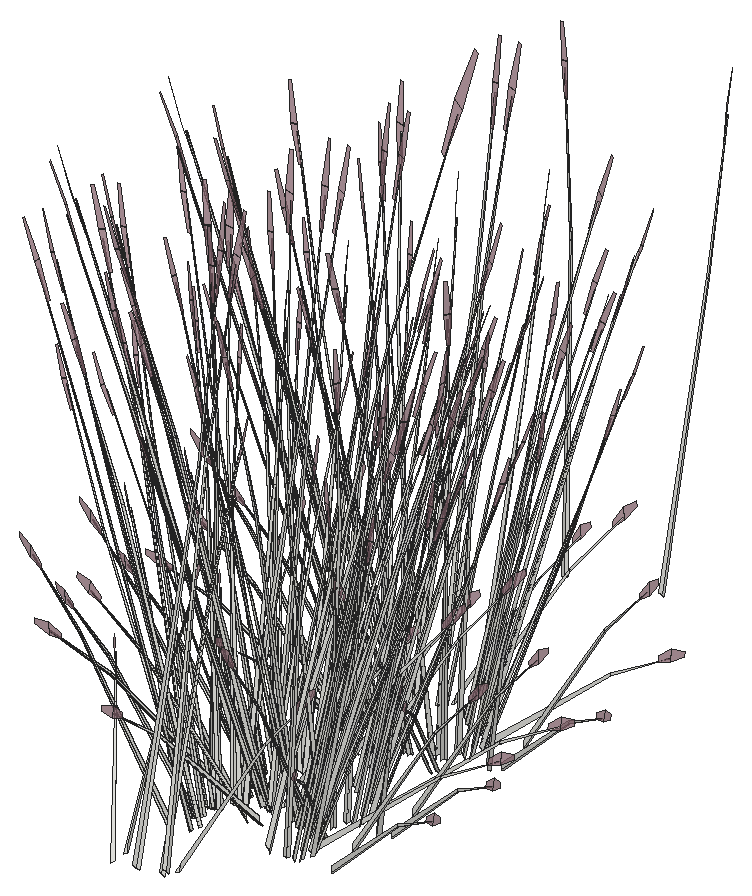
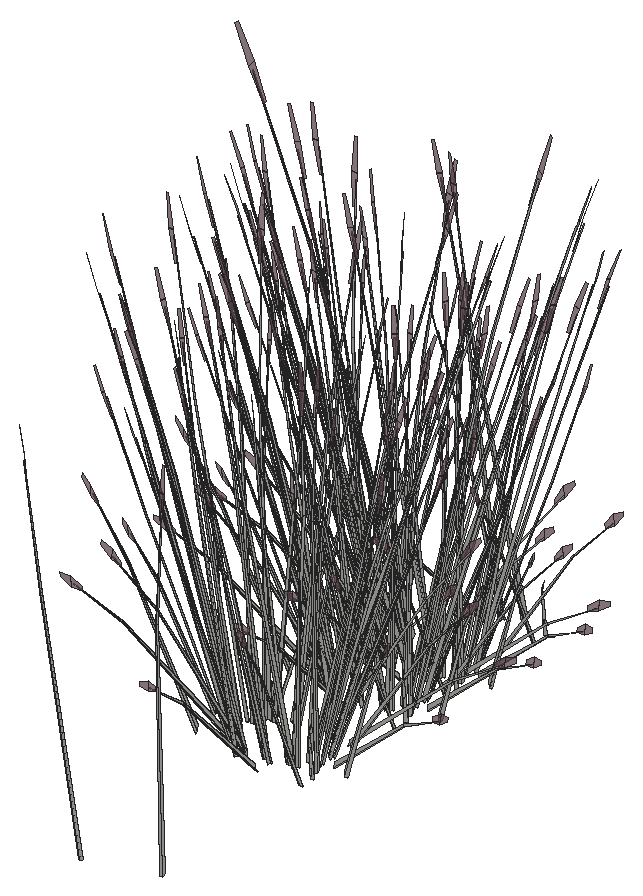
# SketchUp Ruby script. Lengths in inches.
U = 1.inch
M = Sketchup.active_model
def pt(a) = Geom::Point3d.new(a.map { |v| v * U })
def face(e, loops, mat)
  f = e.add_face(loops[0].map { |a| pt(a) })
  loops[1..].each { |l| e.add_face(l.map { |a| pt(a) }).erase! }
  f.material = f.back_material = mat if mat
  f
end
# faces: each face lists its corners as indices into pts; further lists are holes
def faces(e, pts, list, mat = nil) = list.each { |f| face(e, (f[0].is_a?(Array) ? f : [f]).map { |l| l.map { |i| pts[i] } }, mat) }
# xy, xz, yz: faces in a plane at the given z, y or x. An outline is a flat list of corners, or four numbers for a rectangle; further outlines are holes
def ring(l) = l.size == 4 ? [[l[0], l[1]], [l[2], l[1]], [l[2], l[3]], [l[0], l[3]]] : l.each_slice(2).to_a
def flat(e, list, mat, &to3) = list.each { |f| face(e, (f[0].is_a?(Array) ? f : [f]).map { |l| ring(l).map { |u, v| to3.(u, v) } }, mat) }
def xy(e, z, list, mat = nil) = flat(e, list, mat) { |x, y| [x, y, z] }
def xz(e, y, list, mat = nil) = flat(e, list, mat) { |x, z| [x, y, z] }
def yz(e, x, list, mat = nil) = flat(e, list, mat) { |y, z| [x, y, z] }
def lines(e, pts, list) = list.each { |a, b| e.add_line(pt(pts[a]), pt(pts[b])) }
# prism: a flat outline (further loops are holes) pulled along v
def prism(e, loops, v, mat = nil)
  f = face(e, loops, mat); d = Geom::Vector3d.new(v.map { |x| x * U })
  f.pushpull(f.normal.samedirection?(d) ? d.length : -d.length)
end
def box(e, o, s, mat = nil) = prism(e, [[o, [o[0] + s[0], o[1], o[2]], [o[0] + s[0], o[1] + s[1], o[2]], [o[0], o[1] + s[1], o[2]]]], [0, 0, s[2]], mat)
def at(x, y, z, deg = 0) = Geom::Transformation.translation(pt([x, y, z])) * Geom::Transformation.rotation(ORIGIN, Z_AXIS, deg.degrees)
def axes(o, x, y, z) = Geom::Transformation.new([*x, 0, *y, 0, *z, 0, *pt(o).to_a, 1])
def part(name) = M.definitions.add(name)
# library, detail: a bought-in or finely detailed component or shape, given as its bounding box
def library(name, o, s) = part(name).tap { |d| box(d.entities, o, s) }
def detail(e, o, s) = box(e.add_group.entities, o, s)
def put(e, d, t, mat = nil) = e.add_instance(d, t).tap { |i| i.material = mat if mat }
def group(e, t, mat = nil) = e.add_group.tap { |g| g.transformation = t; g.material = mat if mat }.entities
root = M.entities
M.materials.add("LightPink_Translucent").color = [144, 107, 117]
M.materials["LightPink_Translucent"].alpha = 0.75
c1 = part("blade")
p = [[2.15,0.21,22],[0,0.17,0],[0.09,0.45,0],[2.18,0.31,22],[2.29,0.31,22],[0.38,0.45,0],
  [2.48,0.24,33],[2.49,0.24,33],[2.48,0.22,33]]
faces(c1.entities,p,[[0,1,2,3],[4,5,2,3],[6,3,4,7],[8,0,3,6]])
c2 = part("seeds")
p = [[0.3,-0.1,1.38],[-0.01,-0.03,1.59],[-0.01,-0.03,0.03],[0.14,-0.07,-0.07],[0.29,-0.03,3],[0.15,0.01,3.11]]
faces(c2.entities,p,[[0,1,2,3],[1,0,4,5]],"LightPink_Translucent")
c3 = part("blade with seeds")
put(c3.entities,c1,at(0,0,0))
put(c3.entities,c2,axes([2.4,0.25,30.99],[1.5799,-0.05474,1.17369],[-0.12525,1.92788,0.29478],[-0.07173,-0.02425,1.56792]))
put(root,c3,axes([271.4375,361,127.375],[-0.6592,0.22175,0.0643],[-0.32265,-0.40436,0.50621],[0.06366,0.17825,0.77189]))
put(root,c3,axes([267.58,360.37,127.36],[-0.02224,0.12912,1.74944],[0.63107,0.44917,-0.27667],[-0.16521,0.21241,0.14031]))
put(root,c3,axes([269.6,360.08,128.04],[0.98321,0.03233,-0.13498],[-0.02687,0.61208,-0.74919],[-0.0683,0.23574,1.13838]))
put(root,c3,axes([275.86,367.16,127.73],[-0.77872,0.09325,0.35414],[-0.20563,-0.53305,-0.4572],[0.22316,-0.14318,0.87481]))
put(root,c3,axes([271.67,360.96,127.71],[-0.88151,-0.17057,0.53283],[0.30143,-0.56078,0.43934],[0.05297,0.22053,1.10256]))
put(root,c3,axes([276.5625,367.07,127.41],[0.61415,0.2744,0.0643],[-0.35756,0.39076,0.50621],[0.1969,-0.12633,0.77189]))
put(root,c3,axes([276.39,366.96,127.41],[0.22187,0.60049,0.48003],[-0.87033,0.10422,0.3958],[0.25651,-0.14123,0.9933]))
put(root,c3,axes([278.74,367.68,127.39],[0.12414,-0.09938,1.74944],[-0.15889,-0.60963,-0.27667],[0.31148,-0.11559,0.14031]))
put(root,c3,axes([271.98,369.52,127.26],[-0.13683,-0.09148,1.74944],[-0.91315,0.058,-0.27667],[-0.14574,-0.2188,0.14031]))
put(root,c3,axes([268.25,365.3,127.38],[0.06632,0.06511,1.77383],[-0.31973,0.58531,-0.16761],[-0.32381,0.00424,0.31391]))
put(root,c3,axes([267.51,361.69,127.35],[0.10149,-0.03939,1.77383],[0.83886,0.26202,-0.16761],[-0.01971,0.21816,0.31391]))
put(root,c3,axes([269.65,366.32,127.73],[0.50902,0.40851,0.35414],[-0.58122,0.38671,-0.4572],[-0.29531,-0.05884,0.87481]))
put(root,c3,axes([269.51,366.0625,127.71],[-0.0479,0.66354,-0.1216],[-0.90696,-0.01814,-0.67495],[-0.3493,-0.04609,1.02557]))
put(root,c3,axes([276.09,370.64,127.26],[-0.00864,-0.12985,1.74944],[-0.72937,-0.3753,-0.27667],[0.11277,-0.2275,0.14031]))
put(root,c3,axes([275.89,370.17,127.26],[-0.09085,0.04984,1.77383],[-0.89014,-0.16814,-0.16761],[-0.03222,-0.21748,0.31391]))
put(root,c3,axes([276.29,368.61,127.71],[-0.45012,-0.59081,-0.1216],[0.79888,-0.29033,-0.67495],[0.33665,-0.07795,1.02557]))
put(root,c3,axes([271.21,361.96,127.36],[0.1134,0.10507,1.74944],[0.91515,0.04128,-0.27667],[0.09203,0.23172,0.14031]))
put(root,c3,axes([271.05,369.22,127.26],[-0.01669,0.07821,1.77383],[-0.82314,0.28383,-0.16761],[-0.24223,-0.14508,0.31391]))
put(root,c3,axes([270.87,370.61,127.64],[0.99656,-0.1677,0.53763],[0.17295,0.65785,0.4433],[-0.23438,-0.19388,1.11249]))
put(root,c3,axes([273.12,370.73,127.28],[0.88151,0.17057,0.48003],[-0.30143,0.56078,0.3958],[-0.05297,-0.22053,0.9933]))
put(root,c3,axes([275.98,368.43,127.73],[-0.74348,-0.18202,0.35414],[0.21685,-0.53102,-0.4572],[0.29933,-0.04869,0.87481]))
put(root,c3,axes([273.35,370.6875,127.28],[0.6592,-0.22175,0.0643],[0.32265,0.40436,0.50621],[-0.06366,-0.17825,0.77189]))
put(root,c3,axes([268.2,367.46,127.41],[0.25275,-0.59491,0.48003],[0.83094,0.20343,0.3958],[-0.32677,0.03575,0.9933]))
put(root,c3,axes([268.14,367.3,127.41],[-0.32857,-0.44488,0.0643],[0.59916,-0.21775,0.50621],[-0.26412,0.04296,0.77189]))
put(root,c3,axes([271.09,370.75,127.28],[0.4066,-0.41448,0.0643],[0.57901,0.24131,0.50621],[-0.18719,-0.13288,0.77189]))
put(root,c3,axes([273.11,371.14,127.6],[-0.2697,0.50175,0.35414],[-0.78684,-0.14635,-0.4572],[-0.07215,-0.20201,0.87481]))
put(root,c3,axes([275.12,371.35,127.28],[0.63704,0.44518,0.48003],[-0.67652,0.38394,0.3958],[0.11751,-0.20886,0.9933]))
put(root,c3,axes([271.28,370.71,127.98],[-0.59706,0.6255,-0.13619],[-0.86465,-0.36036,-0.75594],[-0.30056,-0.17672,1.14864]))
put(root,c3,axes([275.36,371.4,127.28],[0.73517,0.0304,0.0643],[-0.02016,0.45906,0.50621],[0.07693,-0.17585,0.77189]))
put(root,c3,axes([276.66,368.6,127.41],[0.32857,0.44488,0.0643],[-0.59916,0.21775,0.50621],[0.26412,-0.04296,0.77189]))
put(root,c3,axes([274.81,371.71,127.6],[-0.60531,0.34352,0.35414],[-0.573,-0.39225,-0.4572],[0.08718,-0.19929,0.87481]))
put(root,c3,axes([276.59,368.4375,127.41],[-0.25275,0.59491,0.48003],[-0.83094,-0.20343,0.3958],[0.32677,-0.03575,0.9933]))
put(root,c3,axes([268.81,367.47,127.73],[0.74348,0.18202,0.35414],[-0.21685,0.53102,-0.4572],[-0.29933,0.04869,0.87481]))
put(root,c3,axes([268.99,370.53,127.26],[-0.19249,-0.00461,1.74944],[-0.61281,0.46055,-0.27667],[-0.32697,-0.0941,0.14031]))
put(root,c3,axes([271.22,371.23,127.6],[0.13817,0.52554,0.35414],[-0.78985,0.13877,-0.4572],[-0.21215,-0.1506,0.87481]))
put(root,c3,axes([268.85,371.57,127.64],[0.7388,-0.48151,0.53763],[0.63717,0.51135,0.4433],[-0.34662,-0.08882,1.11249]))
put(root,c3,axes([278.3,372.66,127.26],[-0.11685,-0.00496,1.77383],[-0.48522,-0.53096,-0.16761],[0.19486,-0.17458,0.31391]))
put(root,c3,axes([278.09,370.36,127.38],[-0.08089,-0.05712,1.77383],[0.17695,-0.61228,-0.16761],[0.31864,-0.03912,0.31391]))
put(root,c3,axes([267.56,367.88,127.39],[-0.14609,0.08471,1.74944],[0.01243,0.61893,-0.27667],[-0.33486,0.08049,0.14031]))
put(root,c3,axes([268.5,367.29,127.71],[0.45012,0.59081,-0.1216],[-0.79888,0.29033,-0.67495],[-0.33665,0.07795,1.02557]))
put(root,c3,axes([275.28,369.84,127.71],[0.0479,-0.66354,-0.1216],[0.90696,0.01814,-0.67495],[0.3493,0.04609,1.02557]))
put(root,c3,axes([269.19,371.56,127.28],[0.04505,-0.49615,0.0643],[0.68022,0.0136,0.50621],[-0.26056,-0.05192,0.77189]))
put(root,c3,axes([275.14,369.58,127.73],[-0.50902,-0.40851,0.35414],[0.58122,-0.38671,-0.4572],[0.29531,0.05884,0.87481]))
put(root,c3,axes([275.86,372.77,127.6],[-0.77872,0.09325,0.35414],[-0.20563,-0.53305,-0.4572],[0.22316,-0.14318,0.87481]))
put(root,c3,axes([276.07,369.4375,127.39],[0.19191,-0.01103,1.74944],[0.52639,-0.5069,-0.27667],[0.34136,0.06691,0.14031]))
put(root,c3,axes([268.4,368.94,127.41],[-0.22187,-0.60049,0.48003],[0.87033,-0.10422,0.3958],[-0.25651,0.14123,0.9933]))
put(root,c3,axes([268.23,368.83,127.41],[-0.61415,-0.2744,0.0643],[0.35756,-0.39076,0.50621],[-0.1969,0.12633,0.77189]))
put(root,c3,axes([276.5625,372.68,127.28],[0.61415,0.2744,0.0643],[-0.35756,0.39076,0.50621],[0.1969,-0.12633,0.77189]))
put(root,c3,axes([276.39,372.57,127.28],[0.22187,0.60049,0.48003],[-0.87033,0.10422,0.3958],[0.25651,-0.14123,0.9933]))
put(root,c3,axes([278.74,373.3,127.26],[0.12414,-0.09938,1.74944],[-0.15889,-0.60963,-0.27667],[0.31148,-0.11559,0.14031]))
put(root,c3,axes([268.25,370.92,127.26],[0.06632,0.06511,1.77383],[-0.31973,0.58531,-0.16761],[-0.32381,0.00424,0.31391]))
put(root,c3,axes([268.93,368.74,127.73],[0.77872,-0.09325,0.35414],[0.20563,0.53305,-0.4572],[-0.22316,0.14318,0.87481]))
put(root,c3,axes([265.93,368.51,127.38],[0.11417,0.0175,1.77383],[0.35319,0.57649,-0.16761],[-0.23371,0.15131,0.31391]))
put(root,c3,axes([269.65,371.94,127.6],[0.50902,0.40851,0.35414],[-0.58122,0.38671,-0.4572],[-0.29531,-0.05884,0.87481]))
put(root,c3,axes([275.61,369.95,127.41],[-0.04505,0.49615,0.0643],[-0.68022,-0.0136,0.50621],[0.26056,0.05192,0.77189]))
put(root,c3,axes([275.67,369.79,127.41],[-0.65964,0.42992,0.48003],[-0.5689,-0.45657,0.3958],[0.30948,0.0793,0.9933]))
put(root,c3,axes([267.17,370.26,128.32],[0.78943,0.17416,-0.06488],[-0.24284,0.53604,-0.29416],[-0.12912,0.08139,0.97024]))
put(root,c3,axes([273.57,370.29,127.73],[-0.13817,-0.52554,0.35414],[0.78985,-0.13877,-0.4572],[0.21215,0.1506,0.87481]))
put(root,c3,axes([274.1,367.26,127.15],[-0.77304,-0.33901,1.38283],[0.81626,-0.52782,0.59665],[0.24941,0.31809,1.33663]))
put(root,c3,axes([268.53,368.69,127.71],[0.82753,0.35977,-0.1216],[-0.47675,0.52101,-0.67495],[-0.2338,0.18111,1.02557]))
put(root,c3,axes([273.5,370.56,127.71],[0.53309,-0.55848,-0.1216],[0.77201,0.32175,-0.67495],[0.26836,0.15779,1.02557]))
put(root,c3,axes([275.98,374.04,127.6],[-0.74348,-0.18202,0.35414],[0.21685,-0.53102,-0.4572],[0.29933,-0.04869,0.87481]))
put(root,c3,axes([268.2,373.07,127.28],[0.25275,-0.59491,0.48003],[0.83094,0.20343,0.3958],[-0.32677,0.03575,0.9933]))
put(root,c3,axes([269.98,369.8,127.73],[0.60531,-0.34352,0.35414],[0.573,0.39225,-0.4572],[-0.08718,0.19929,0.87481]))
put(root,c3,axes([268.14,372.92,127.28],[-0.32857,-0.44488,0.0643],[0.59916,-0.21775,0.50621],[-0.26412,0.04296,0.77189]))
put(root,c3,axes([272.8,371.02,127.38],[0.00265,-0.07899,1.77383],[0.76665,-0.34851,-0.16761],[0.2663,0.12439,0.31391]))
put(root,c3,axes([269.4375,370.12,127.41],[-0.73517,-0.0304,0.0643],[0.02016,-0.45906,0.50621],[-0.07693,0.17585,0.77189]))
put(root,c3,axes([269.67,370.16,127.41],[-0.63704,-0.44518,0.48003],[0.67652,-0.38394,0.3958],[-0.11751,0.20886,0.9933]))
put(root,c3,axes([271.68,370.37,127.73],[0.2697,-0.50175,0.35414],[0.78684,0.14635,-0.4572],[0.07215,0.20201,0.87481]))
put(root,c3,axes([273.7,370.76,127.41],[-0.4066,0.41448,0.0643],[-0.57901,-0.24131,0.50621],[0.18719,0.13288,0.77189]))
put(root,c3,axes([272.74,372.16,128.32],[0.61821,-0.37431,-0.06488],[0.56645,0.40995,-0.29416],[0.03988,0.11616,0.97024]))
put(root,c3,axes([273.87,370.65,127.41],[-0.88979,0.14973,0.48003],[-0.15442,-0.58737,0.3958],[0.20926,0.17311,0.9933]))
put(root,c3,axes([276.66,374.21,127.28],[0.32857,0.44488,0.0643],[-0.59916,0.21775,0.50621],[0.26412,-0.04296,0.77189]))
put(root,c3,axes([276.59,374.05,127.28],[-0.25275,0.59491,0.48003],[-0.83094,-0.20343,0.3958],[0.32677,-0.03575,0.9933]))
put(root,c3,axes([271.4375,370.82,127.41],[-0.6592,0.22175,0.0643],[-0.32265,-0.40436,0.50621],[0.06366,0.17825,0.77189]))
put(root,c3,axes([267.58,370.19,127.39],[-0.02224,0.12912,1.74944],[0.63107,0.44917,-0.27667],[-0.16521,0.21241,0.14031]))
put(root,c3,axes([268.81,373.08,127.6],[0.74348,0.18202,0.35414],[-0.21685,0.53102,-0.4572],[-0.29933,0.04869,0.87481]))
put(root,c3,axes([269.6,369.9,128.07],[0.98321,0.03233,-0.13498],[-0.02687,0.61208,-0.74919],[-0.0683,0.23574,1.13838]))
put(root,c3,axes([271.42,370.58,127.71],[0.87543,-0.30377,-0.1216],[0.4302,0.53915,-0.67495],[0.1155,0.2272,1.02557]))
put(root,c3,axes([271.67,370.78,127.74],[-0.88151,-0.17057,0.53283],[0.30143,-0.56078,0.43934],[0.05297,0.22053,1.10256]))
put(root,c3,axes([278.09,375.98,127.26],[-0.08089,-0.05712,1.77383],[0.17695,-0.61228,-0.16761],[0.31864,-0.03912,0.31391]))
put(root,c3,axes([267.56,373.49,127.26],[-0.14609,0.08471,1.74944],[0.01243,0.61893,-0.27667],[-0.33486,0.08049,0.14031]))
put(root,c3,axes([267.51,371.51,127.38],[0.10149,-0.03939,1.77383],[0.83886,0.26202,-0.16761],[-0.01971,0.21816,0.31391]))
put(root,c3,axes([275.14,375.1875,127.6],[-0.50902,-0.40851,0.35414],[0.58122,-0.38671,-0.4572],[0.29531,0.05884,0.87481]))
put(root,c3,axes([271.98,379.88,127.3],[-0.13683,-0.09148,1.74944],[-0.91315,0.058,-0.27667],[-0.14574,-0.2188,0.14031]))
put(root,c3,axes([276.07,375.05,127.26],[0.19191,-0.01103,1.74944],[0.52639,-0.5069,-0.27667],[0.34136,0.06691,0.14031]))
put(root,c3,axes([271.21,371.79,127.39],[0.1134,0.10507,1.74944],[0.91515,0.04128,-0.27667],[0.09203,0.23172,0.14031]))
put(root,c3,axes([268.4,374.56,127.28],[-0.22187,-0.60049,0.48003],[0.87033,-0.10422,0.3958],[-0.25651,0.14123,0.9933]))
put(root,c3,axes([268.23,374.44,127.28],[-0.61415,-0.2744,0.0643],[0.35756,-0.39076,0.50621],[-0.1969,0.12633,0.77189]))
put(root,c3,axes([276.09,381,127.3],[-0.00864,-0.12985,1.74944],[-0.72937,-0.3753,-0.27667],[0.11277,-0.2275,0.14031]))
put(root,c3,axes([275.89,380.54,127.29],[-0.09085,0.04984,1.77383],[-0.89014,-0.16814,-0.16761],[-0.03222,-0.21748,0.31391]))
put(root,c3,axes([268.93,374.36,127.6],[0.77872,-0.09325,0.35414],[0.20563,0.53305,-0.4572],[-0.22316,0.14318,0.87481]))
put(root,c3,axes([265.93,374.12,127.26],[0.11417,0.0175,1.77383],[0.35319,0.57649,-0.16761],[-0.23371,0.15131,0.31391]))
put(root,c3,axes([271.05,379.58,127.29],[-0.01669,0.07821,1.77383],[-0.82314,0.28383,-0.16761],[-0.24223,-0.14508,0.31391]))
put(root,c3,axes([275.61,375.56,127.28],[-0.04505,0.49615,0.0643],[-0.68022,-0.0136,0.50621],[0.26056,0.05192,0.77189]))
put(root,c3,axes([270.87,380.97,127.67],[0.99656,-0.1677,0.53763],[0.17295,0.65785,0.4433],[-0.23438,-0.19388,1.11249]))
put(root,c3,axes([275.67,375.4,127.28],[-0.65964,0.42992,0.48003],[-0.5689,-0.45657,0.3958],[0.30948,0.0793,0.9933]))
put(root,c3,axes([273.12,381.09,127.3125],[0.88151,0.17057,0.48003],[-0.30143,0.56078,0.3958],[-0.05297,-0.22053,0.9933]))
put(root,c3,axes([273.35,381.05,127.3125],[0.6592,-0.22175,0.0643],[0.32265,0.40436,0.50621],[-0.06366,-0.17825,0.77189]))
put(root,c3,axes([267.17,375.87,128.19],[0.78943,0.17416,-0.06488],[-0.24284,0.53604,-0.29416],[-0.12912,0.08139,0.97024]))
put(root,c3,axes([273.57,375.9,127.6],[-0.13817,-0.52554,0.35414],[0.78985,-0.13877,-0.4572],[0.21215,0.1506,0.87481]))
put(root,c3,axes([271.09,381.11,127.3125],[0.4066,-0.41448,0.0643],[0.57901,0.24131,0.50621],[-0.18719,-0.13288,0.77189]))
put(root,c3,axes([273.11,381.5,127.63],[-0.2697,0.50175,0.35414],[-0.78684,-0.14635,-0.4572],[-0.07215,-0.20201,0.87481]))
put(root,c3,axes([269.98,375.42,127.6],[0.60531,-0.34352,0.35414],[0.573,0.39225,-0.4572],[-0.08718,0.19929,0.87481]))
put(root,c3,axes([275.12,381.72,127.3125],[0.63704,0.44518,0.48003],[-0.67652,0.38394,0.3958],[0.11751,-0.20886,0.9933]))
put(root,c3,axes([271.28,381.07,128.01],[-0.59706,0.6255,-0.13619],[-0.86465,-0.36036,-0.75594],[-0.30056,-0.17672,1.14864]))
put(root,c3,axes([272.8,376.63,127.26],[0.00265,-0.07899,1.77383],[0.76665,-0.34851,-0.16761],[0.2663,0.12439,0.31391]))
put(root,c3,axes([275.36,381.76,127.3125],[0.73517,0.0304,0.0643],[-0.02016,0.45906,0.50621],[0.07693,-0.17585,0.77189]))
put(root,c3,axes([269.4375,375.73,127.28],[-0.73517,-0.0304,0.0643],[0.02016,-0.45906,0.50621],[-0.07693,0.17585,0.77189]))
put(root,c3,axes([269.67,375.77,127.28],[-0.63704,-0.44518,0.48003],[0.67652,-0.38394,0.3958],[-0.11751,0.20886,0.9933]))
put(root,c3,axes([274.81,382.07,127.63],[-0.60531,0.34352,0.35414],[-0.573,-0.39225,-0.4572],[0.08718,-0.19929,0.87481]))
put(root,c3,axes([271.68,375.98,127.6],[0.2697,-0.50175,0.35414],[0.78684,0.14635,-0.4572],[0.07215,0.20201,0.87481]))
put(root,c3,axes([268.99,380.89,127.3],[-0.19249,-0.00461,1.74944],[-0.61281,0.46055,-0.27667],[-0.32697,-0.0941,0.14031]))
put(root,c3,axes([273.7,376.375,127.28],[-0.4066,0.41448,0.0643],[-0.57901,-0.24131,0.50621],[0.18719,0.13288,0.77189]))
put(root,c3,axes([272.74,377.77,128.19],[0.61821,-0.37431,-0.06488],[0.56645,0.40995,-0.29416],[0.03988,0.11616,0.97024]))
put(root,c3,axes([273.87,376.26,127.28],[-0.88979,0.14973,0.48003],[-0.15442,-0.58737,0.3958],[0.20926,0.17311,0.9933]))
put(root,c3,axes([271.22,381.59,127.63],[0.13817,0.52554,0.35414],[-0.78985,0.13877,-0.4572],[-0.21215,-0.1506,0.87481]))
put(root,c3,axes([268.85,381.93,127.67],[0.7388,-0.48151,0.53763],[0.63717,0.51135,0.4433],[-0.34662,-0.08882,1.11249]))
put(root,c3,axes([278.3,383.02,127.29],[-0.11685,-0.00496,1.77383],[-0.48522,-0.53096,-0.16761],[0.19486,-0.17458,0.31391]))
put(root,c3,axes([271.4375,376.4375,127.28],[-0.6592,0.22175,0.0643],[-0.32265,-0.40436,0.50621],[0.06366,0.17825,0.77189]))
put(root,c3,axes([267.58,375.8,127.26],[-0.02224,0.12912,1.74944],[0.63107,0.44917,-0.27667],[-0.16521,0.21241,0.14031]))
put(root,c3,axes([269.6,375.51,127.95],[0.98321,0.03233,-0.13498],[-0.02687,0.61208,-0.74919],[-0.0683,0.23574,1.13838]))
put(root,c3,axes([271.67,376.39,127.61],[-0.88151,-0.17057,0.53283],[0.30143,-0.56078,0.43934],[0.05297,0.22053,1.10256]))
put(root,c3,axes([269.19,381.93,127.3125],[0.04505,-0.49615,0.0643],[0.68022,0.0136,0.50621],[-0.26056,-0.05192,0.77189]))
put(root,c3,axes([275.86,383.13,127.63],[-0.77872,0.09325,0.35414],[-0.20563,-0.53305,-0.4572],[0.22316,-0.14318,0.87481]))
put(root,c3,axes([267.51,377.125,127.26],[0.10149,-0.03939,1.77383],[0.83886,0.26202,-0.16761],[-0.01971,0.21816,0.31391]))
put(root,c3,axes([276.5625,383.05,127.3125],[0.61415,0.2744,0.0643],[-0.35756,0.39076,0.50621],[0.1969,-0.12633,0.77189]))
put(root,c3,axes([276.39,382.93,127.3125],[0.22187,0.60049,0.48003],[-0.87033,0.10422,0.3958],[0.25651,-0.14123,0.9933]))
put(root,c3,axes([278.74,383.66,127.3],[0.12414,-0.09938,1.74944],[-0.15889,-0.60963,-0.27667],[0.31148,-0.11559,0.14031]))
put(root,c3,axes([268.25,381.28,127.29],[0.06632,0.06511,1.77383],[-0.31973,0.58531,-0.16761],[-0.32381,0.00424,0.31391]))
put(root,c3,axes([271.21,377.4,127.26],[0.1134,0.10507,1.74944],[0.91515,0.04128,-0.27667],[0.09203,0.23172,0.14031]))
put(root,c3,axes([269.65,382.3,127.63],[0.50902,0.40851,0.35414],[-0.58122,0.38671,-0.4572],[-0.29531,-0.05884,0.87481]))
put(root,c3,axes([275.98,384.41,127.63],[-0.74348,-0.18202,0.35414],[0.21685,-0.53102,-0.4572],[0.29933,-0.04869,0.87481]))
put(root,c3,axes([268.2,383.4375,127.3125],[0.25275,-0.59491,0.48003],[0.83094,0.20343,0.3958],[-0.32677,0.03575,0.9933]))
put(root,c3,axes([268.14,383.28,127.3125],[-0.32857,-0.44488,0.0643],[0.59916,-0.21775,0.50621],[-0.26412,0.04296,0.77189]))
put(root,c3,axes([276.66,384.57,127.3125],[0.32857,0.44488,0.0643],[-0.59916,0.21775,0.50621],[0.26412,-0.04296,0.77189]))
put(root,c3,axes([276.59,384.41,127.3125],[-0.25275,0.59491,0.48003],[-0.83094,-0.20343,0.3958],[0.32677,-0.03575,0.9933]))
put(root,c3,axes([268.81,383.44,127.63],[0.74348,0.18202,0.35414],[-0.21685,0.53102,-0.4572],[-0.29933,0.04869,0.87481]))
put(root,c3,axes([278.09,386.34,127.29],[-0.08089,-0.05712,1.77383],[0.17695,-0.61228,-0.16761],[0.31864,-0.03912,0.31391]))
put(root,c3,axes([267.56,383.85,127.3],[-0.14609,0.08471,1.74944],[0.01243,0.61893,-0.27667],[-0.33486,0.08049,0.14031]))
put(root,c3,axes([275.14,385.55,127.63],[-0.50902,-0.40851,0.35414],[0.58122,-0.38671,-0.4572],[0.29531,0.05884,0.87481]))
put(root,c3,axes([276.07,385.41,127.3],[0.19191,-0.01103,1.74944],[0.52639,-0.5069,-0.27667],[0.34136,0.06691,0.14031]))
put(root,c3,axes([268.4,384.92,127.3125],[-0.22187,-0.60049,0.48003],[0.87033,-0.10422,0.3958],[-0.25651,0.14123,0.9933]))
put(root,c3,axes([268.23,384.8,127.3125],[-0.61415,-0.2744,0.0643],[0.35756,-0.39076,0.50621],[-0.1969,0.12633,0.77189]))
put(root,c3,axes([268.93,384.72,127.63],[0.77872,-0.09325,0.35414],[0.20563,0.53305,-0.4572],[-0.22316,0.14318,0.87481]))
put(root,c3,axes([265.93,384.48,127.29],[0.11417,0.0175,1.77383],[0.35319,0.57649,-0.16761],[-0.23371,0.15131,0.31391]))
put(root,c3,axes([275.61,385.92,127.3125],[-0.04505,0.49615,0.0643],[-0.68022,-0.0136,0.50621],[0.26056,0.05192,0.77189]))
put(root,c3,axes([275.67,385.76,127.3125],[-0.65964,0.42992,0.48003],[-0.5689,-0.45657,0.3958],[0.30948,0.0793,0.9933]))
put(root,c3,axes([267.17,386.23,128.23],[0.78943,0.17416,-0.06488],[-0.24284,0.53604,-0.29416],[-0.12912,0.08139,0.97024]))
put(root,c3,axes([273.57,386.26,127.63],[-0.13817,-0.52554,0.35414],[0.78985,-0.13877,-0.4572],[0.21215,0.1506,0.87481]))
put(root,c3,axes([269.98,385.78,127.63],[0.60531,-0.34352,0.35414],[0.573,0.39225,-0.4572],[-0.08718,0.19929,0.87481]))
put(root,c3,axes([272.8,387,127.29],[0.00265,-0.07899,1.77383],[0.76665,-0.34851,-0.16761],[0.2663,0.12439,0.31391]))
put(root,c3,axes([269.4375,386.09,127.3125],[-0.73517,-0.0304,0.0643],[0.02016,-0.45906,0.50621],[-0.07693,0.17585,0.77189]))
put(root,c3,axes([269.67,386.13,127.3125],[-0.63704,-0.44518,0.48003],[0.67652,-0.38394,0.3958],[-0.11751,0.20886,0.9933]))
put(root,c3,axes([271.68,386.34,127.63],[0.2697,-0.50175,0.35414],[0.78684,0.14635,-0.4572],[0.07215,0.20201,0.87481]))
put(root,c3,axes([273.7,386.74,127.3125],[-0.4066,0.41448,0.0643],[-0.57901,-0.24131,0.50621],[0.18719,0.13288,0.77189]))
put(root,c3,axes([272.74,388.13,128.23],[0.61821,-0.37431,-0.06488],[0.56645,0.40995,-0.29416],[0.03988,0.11616,0.97024]))
put(root,c3,axes([273.87,386.62,127.3125],[-0.88979,0.14973,0.48003],[-0.15442,-0.58737,0.3958],[0.20926,0.17311,0.9933]))
put(root,c3,axes([271.4375,386.8,127.3125],[-0.6592,0.22175,0.0643],[-0.32265,-0.40436,0.50621],[0.06366,0.17825,0.77189]))
put(root,c3,axes([267.58,386.17,127.3],[-0.02224,0.12912,1.74944],[0.63107,0.44917,-0.27667],[-0.16521,0.21241,0.14031]))
put(root,c3,axes([269.6,385.875,127.98],[0.98321,0.03233,-0.13498],[-0.02687,0.61208,-0.74919],[-0.0683,0.23574,1.13838]))
put(root,c3,axes([271.67,386.76,127.64],[-0.88151,-0.17057,0.53283],[0.30143,-0.56078,0.43934],[0.05297,0.22053,1.10256]))
put(root,c3,axes([267.51,387.49,127.29],[0.10149,-0.03939,1.77383],[0.83886,0.26202,-0.16761],[-0.01971,0.21816,0.31391]))
put(root,c3,axes([271.21,387.76,127.3],[0.1134,0.10507,1.74944],[0.91515,0.04128,-0.27667],[0.09203,0.23172,0.14031]))
put(root,c3,axes([267.17,403.34,127.5625],[0.78943,0.17416,-0.06488],[-0.24284,0.53604,-0.29416],[-0.12912,0.08139,0.97024]))
put(root,c3,axes([272.74,405.25,127.5625],[0.61821,-0.37431,-0.06488],[0.56645,0.40995,-0.29416],[0.03988,0.11616,0.97024]))
